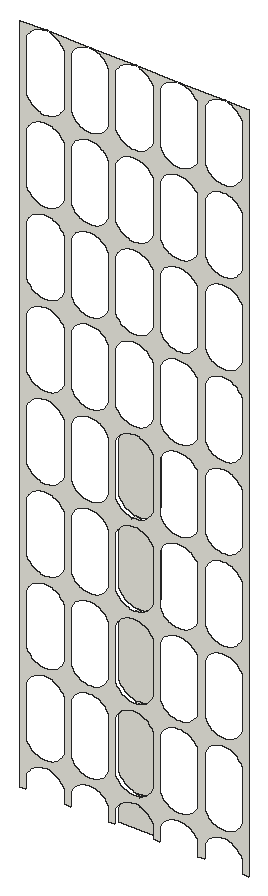
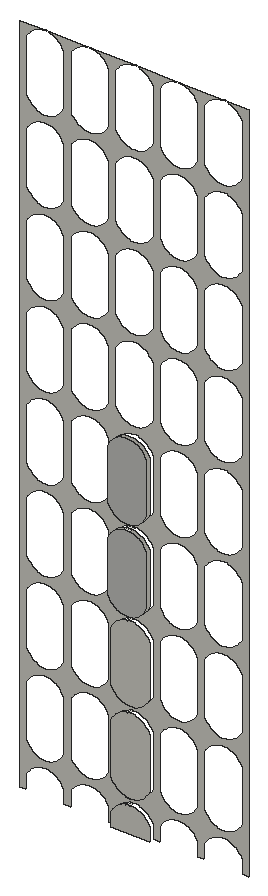
# SketchUp Ruby script. Lengths in inches.
U = 1.inch
M = Sketchup.active_model
def pt(a) = Geom::Point3d.new(a.map { |v| v * U })
def face(e, loops, mat)
  f = e.add_face(loops[0].map { |a| pt(a) })
  loops[1..].each { |l| e.add_face(l.map { |a| pt(a) }).erase! }
  f.material = f.back_material = mat if mat
  f
end
# faces: each face lists its corners as indices into pts; further lists are holes
def faces(e, pts, list, mat = nil) = list.each { |f| face(e, (f[0].is_a?(Array) ? f : [f]).map { |l| l.map { |i| pts[i] } }, mat) }
# xy, xz, yz: faces in a plane at the given z, y or x. An outline is a flat list of corners, or four numbers for a rectangle; further outlines are holes
def ring(l) = l.size == 4 ? [[l[0], l[1]], [l[2], l[1]], [l[2], l[3]], [l[0], l[3]]] : l.each_slice(2).to_a
def flat(e, list, mat, &to3) = list.each { |f| face(e, (f[0].is_a?(Array) ? f : [f]).map { |l| ring(l).map { |u, v| to3.(u, v) } }, mat) }
def xy(e, z, list, mat = nil) = flat(e, list, mat) { |x, y| [x, y, z] }
def xz(e, y, list, mat = nil) = flat(e, list, mat) { |x, z| [x, y, z] }
def yz(e, x, list, mat = nil) = flat(e, list, mat) { |y, z| [x, y, z] }
def lines(e, pts, list) = list.each { |a, b| e.add_line(pt(pts[a]), pt(pts[b])) }
# prism: a flat outline (further loops are holes) pulled along v
def prism(e, loops, v, mat = nil)
  f = face(e, loops, mat); d = Geom::Vector3d.new(v.map { |x| x * U })
  f.pushpull(f.normal.samedirection?(d) ? d.length : -d.length)
end
def box(e, o, s, mat = nil) = prism(e, [[o, [o[0] + s[0], o[1], o[2]], [o[0] + s[0], o[1] + s[1], o[2]], [o[0], o[1] + s[1], o[2]]]], [0, 0, s[2]], mat)
def at(x, y, z, deg = 0) = Geom::Transformation.translation(pt([x, y, z])) * Geom::Transformation.rotation(ORIGIN, Z_AXIS, deg.degrees)
def axes(o, x, y, z) = Geom::Transformation.new([*x, 0, *y, 0, *z, 0, *pt(o).to_a, 1])
def part(name) = M.definitions.add(name)
# library, detail: a bought-in or finely detailed component or shape, given as its bounding box
def library(name, o, s) = part(name).tap { |d| box(d.entities, o, s) }
def detail(e, o, s) = box(e.add_group.entities, o, s)
def put(e, d, t, mat = nil) = e.add_instance(d, t).tap { |i| i.material = mat if mat }
def group(e, t, mat = nil) = e.add_group.tap { |g| g.transformation = t; g.material = mat if mat }.entities
root = M.entities
M.materials.add("Tafisa-Gardenia-or-Gardenia-PM775-4K").color = [246, 245, 235]
xz(root,138,[[[64.5,6,65.5,6,65.5,8,65.637,8.288,65.801,8.56,65.991,8.816,66.205,9.051,66.441,9.265,66.697,9.454,66.97,9.618,67.258,9.753,67.558,9.861,67.867,9.938,68.182,9.984,68.5,10,68.818,9.984,69.133,9.938,69.442,9.861,69.742,9.753,70.03,9.618,70.303,9.454,70.559,9.265,70.795,9.051,71.009,8.816,71.199,8.56,71.363,8.288,71.5,8,71.5,6,72.5,6,72.5,8,72.637,8.288,72.801,8.56,72.991,8.816,73.205,9.051,73.441,9.265,73.697,9.454,73.97,9.618,74.258,9.753,74.558,9.861,74.867,9.938,75.182,9.984,75.5,10,75.818,9.984,76.133,9.938,76.442,9.861,76.742,9.753,77.03,9.618,77.303,9.454,77.559,9.265,77.795,9.051,78.009,8.816,78.199,8.56,78.363,8.288,78.5,8,78.5,6,79.5,6,79.5,8,79.637,8.288,79.801,8.56,79.991,8.816,80.205,9.051,80.441,9.265,80.697,9.454,80.97,9.618,81.258,9.753,81.558,9.861,81.867,9.938,82.182,9.984,82.5,10,82.818,9.984,83.133,9.938,83.442,9.861,83.742,9.753,84.03,9.618,84.303,9.454,84.559,9.265,84.795,9.051,85.009,8.816,85.199,8.56,85.363,8.288,85.5,8,85.5,6,86.5,6,86.5,8,86.64,8.288,86.808,8.561,87.001,8.817,87.218,9.052,87.457,9.266,87.715,9.455,87.991,9.618,88.281,9.754,88.583,9.861,88.894,9.938,89.211,9.984,89.531,10,89.851,9.984,90.168,9.938,90.479,9.861,90.781,9.754,91.071,9.618,91.347,9.455,91.606,9.266,91.845,9.052,92.062,8.817,92.255,8.561,92.422,8.288,92.5625,8,92.5625,6,93.5625,6,93.5625,8,93.696,8.287,93.857,8.559,94.043,8.815,94.255,9.05,94.488,9.264,94.741,9.453,95.012,9.617,95.298,9.753,95.596,9.86,95.902,9.9375,96.215,9.984,96.531,10,96.847,9.984,97.16,9.9375,97.467,9.86,97.765,9.753,98.05,9.617,98.321,9.453,98.574,9.264,98.808,9.05,99.019,8.815,99.206,8.559,99.367,8.287,99.5,8,99.5,6,100.5,6,100.5,114,96.531,114,96.847,113.984,97.16,113.9375,97.467,113.86,97.765,113.753,98.05,113.617,98.321,113.453,98.574,113.264,98.808,113.05,99.019,112.815,99.206,112.559,99.367,112.287,99.5,112,99.5,104,99.367,103.713,99.206,103.441,99.019,103.185,98.808,102.95,98.574,102.736,98.321,102.547,98.05,102.383,97.765,102.247,97.467,102.14,97.16,102.0625,96.847,102.016,96.531,102,96.215,102.016,95.902,102.0625,95.596,102.14,95.298,102.247,95.012,102.383,94.741,102.547,94.488,102.736,94.255,102.95,94.043,103.185,93.857,103.441,93.696,103.713,93.5625,104,93.5625,112,93.696,112.287,93.857,112.559,94.043,112.815,94.255,113.05,94.488,113.264,94.741,113.453,95.012,113.617,95.298,113.753,95.596,113.86,95.902,113.9375,96.215,113.984,96.531,114,89.531,114,89.851,113.984,90.168,113.938,90.479,113.861,90.781,113.754,91.071,113.618,91.347,113.455,91.606,113.266,91.845,113.052,92.062,112.817,92.255,112.561,92.422,112.288,92.5625,112,92.5625,104,92.422,103.712,92.255,103.439,92.062,103.183,91.845,102.948,91.606,102.734,91.347,102.545,91.071,102.382,90.781,102.246,90.479,102.139,90.168,102.062,89.851,102.016,89.531,102,89.211,102.016,88.894,102.062,88.583,102.139,88.281,102.246,87.991,102.382,87.715,102.545,87.457,102.734,87.218,102.948,87.001,103.183,86.808,103.439,86.64,103.712,86.5,104,86.5,112,86.64,112.288,86.808,112.561,87.001,112.817,87.218,113.052,87.457,113.266,87.715,113.455,87.991,113.618,88.281,113.754,88.583,113.861,88.894,113.938,89.211,113.984,89.531,114,82.5,114,82.818,113.984,83.133,113.938,83.442,113.861,83.742,113.753,84.03,113.618,84.303,113.454,84.559,113.265,84.795,113.051,85.009,112.816,85.199,112.56,85.363,112.288,85.5,112,85.5,104,85.363,103.712,85.199,103.44,85.009,103.184,84.795,102.949,84.559,102.735,84.303,102.546,84.03,102.382,83.742,102.247,83.442,102.139,83.133,102.062,82.818,102.016,82.5,102,82.182,102.016,81.867,102.062,81.558,102.139,81.258,102.247,80.97,102.382,80.697,102.546,80.441,102.735,80.205,102.949,79.991,103.184,79.801,103.44,79.637,103.712,79.5,104,79.5,112,79.637,112.288,79.801,112.56,79.991,112.816,80.205,113.051,80.441,113.265,80.697,113.454,80.97,113.618,81.258,113.753,81.558,113.861,81.867,113.938,82.182,113.984,82.5,114,75.5,114,75.818,113.984,76.133,113.938,76.442,113.861,76.742,113.753,77.03,113.618,77.303,113.454,77.559,113.265,77.795,113.051,78.009,112.816,78.199,112.56,78.363,112.288,78.5,112,78.5,104,78.363,103.712,78.199,103.44,78.009,103.184,77.795,102.949,77.559,102.735,77.303,102.546,77.03,102.382,76.742,102.247,76.442,102.139,76.133,102.062,75.818,102.016,75.5,102,75.182,102.016,74.867,102.062,74.558,102.139,74.258,102.247,73.97,102.382,73.697,102.546,73.441,102.735,73.205,102.949,72.991,103.184,72.801,103.44,72.637,103.712,72.5,104,72.5,112,72.637,112.288,72.801,112.56,72.991,112.816,73.205,113.051,73.441,113.265,73.697,113.454,73.97,113.618,74.258,113.753,74.558,113.861,74.867,113.938,75.182,113.984,75.5,114,68.5,114,68.818,113.984,69.133,113.938,69.442,113.861,69.742,113.753,70.03,113.618,70.303,113.454,70.559,113.265,70.795,113.051,71.009,112.816,71.199,112.56,71.363,112.288,71.5,112,71.5,104,71.363,103.712,71.199,103.44,71.009,103.184,70.795,102.949,70.559,102.735,70.303,102.546,70.03,102.382,69.742,102.247,69.442,102.139,69.133,102.062,68.818,102.016,68.5,102,68.182,102.016,67.867,102.062,67.558,102.139,67.258,102.247,66.97,102.382,66.697,102.546,66.441,102.735,66.205,102.949,65.991,103.184,65.801,103.44,65.637,103.712,65.5,104,65.5,112,65.637,112.288,65.801,112.56,65.991,112.816,66.205,113.051,66.441,113.265,66.697,113.454,66.97,113.618,67.258,113.753,67.558,113.861,67.867,113.938,68.182,113.984,68.5,114,64.5,114],[89.531,89,89.211,89.016,88.894,89.062,88.583,89.139,88.281,89.246,87.991,89.382,87.715,89.545,87.457,89.734,87.218,89.948,87.001,90.183,86.808,90.439,86.64,90.712,86.5,91,86.5,99,86.64,99.288,86.808,99.561,87.001,99.817,87.218,100.052,87.457,100.266,87.715,100.455,87.991,100.618,88.281,100.754,88.583,100.861,88.894,100.938,89.211,100.984,89.531,101,89.851,100.984,90.168,100.938,90.479,100.861,90.781,100.754,91.071,100.618,91.347,100.455,91.606,100.266,91.845,100.052,92.062,99.817,92.255,99.561,92.422,99.288,92.5625,99,92.5625,91,92.422,90.712,92.255,90.439,92.062,90.183,91.845,89.948,91.606,89.734,91.347,89.545,91.071,89.382,90.781,89.246,90.479,89.139,90.168,89.062,89.851,89.016],[89.531,11,89.211,11.016,88.894,11.062,88.583,11.139,88.281,11.246,87.991,11.382,87.715,11.545,87.457,11.734,87.218,11.948,87.001,12.183,86.808,12.439,86.64,12.712,86.5,13,86.5,21,86.64,21.288,86.808,21.561,87.001,21.817,87.218,22.052,87.457,22.266,87.715,22.455,87.991,22.618,88.281,22.754,88.583,22.861,88.894,22.938,89.016,22.956,89.211,22.984,89.531,23,89.851,22.984,90.168,22.938,90.479,22.861,90.781,22.754,91.071,22.618,91.347,22.455,91.606,22.266,91.845,22.052,92.062,21.817,92.255,21.561,92.422,21.288,92.5625,21,92.5625,13,92.422,12.712,92.255,12.439,92.062,12.183,91.845,11.948,91.606,11.734,91.347,11.545,91.071,11.382,90.781,11.246,90.479,11.139,90.168,11.062,89.851,11.016],[89.531,24,89.211,24.016,89.016,24.044,88.894,24.062,88.583,24.139,88.281,24.246,87.991,24.382,87.715,24.545,87.457,24.734,87.218,24.948,87.001,25.183,86.808,25.439,86.64,25.712,86.5,26,86.5,34,86.64,34.288,86.808,34.561,86.863,34.634,87.001,34.817,87.218,35.052,87.457,35.266,87.715,35.455,87.991,35.618,88.281,35.754,88.583,35.861,88.894,35.938,89.016,35.956,89.211,35.984,89.531,36,89.851,35.984,90.168,35.938,90.479,35.861,90.781,35.754,91.071,35.618,91.347,35.455,91.606,35.266,91.845,35.052,92.062,34.817,92.255,34.561,92.422,34.288,92.5625,34,92.5625,26,92.422,25.712,92.255,25.439,92.062,25.183,91.845,24.948,91.606,24.734,91.347,24.545,91.071,24.382,90.781,24.246,90.479,24.139,90.168,24.062,89.851,24.016],[89.531,76,89.211,76.016,89.016,76.044,88.894,76.062,88.583,76.139,88.281,76.246,87.991,76.382,87.715,76.545,87.457,76.734,87.218,76.948,87.001,77.183,86.808,77.439,86.64,77.712,86.5,78,86.5,86,86.64,86.288,86.808,86.561,87.001,86.817,87.218,87.052,87.457,87.266,87.715,87.455,87.991,87.618,88.281,87.754,88.583,87.861,88.894,87.938,89.211,87.984,89.531,88,89.851,87.984,90.168,87.938,90.479,87.861,90.781,87.754,91.071,87.618,91.347,87.455,91.606,87.266,91.845,87.052,92.062,86.817,92.255,86.561,92.422,86.288,92.5625,86,92.5625,78,92.422,77.712,92.255,77.439,92.062,77.183,91.845,76.948,91.606,76.734,91.347,76.545,91.071,76.382,90.781,76.246,90.479,76.139,90.168,76.062,89.851,76.016],[89.531,63,89.211,63.016,89.016,63.044,88.894,63.062,88.782,63.09,88.583,63.139,88.281,63.246,87.991,63.382,87.715,63.545,87.457,63.734,87.218,63.948,87.001,64.183,86.808,64.439,86.64,64.712,86.5,65,86.5,73,86.64,73.288,86.808,73.561,87.001,73.817,87.218,74.052,87.457,74.266,87.715,74.455,87.991,74.618,88.281,74.754,88.583,74.861,88.894,74.938,89.016,74.956,89.211,74.984,89.531,75,89.851,74.984,90.168,74.938,90.479,74.861,90.781,74.754,91.071,74.618,91.347,74.455,91.606,74.266,91.845,74.052,92.062,73.817,92.255,73.561,92.422,73.288,92.5625,73,92.5625,65,92.422,64.712,92.255,64.439,92.062,64.183,91.845,63.948,91.606,63.734,91.347,63.545,91.071,63.382,90.781,63.246,90.479,63.139,90.168,63.062,89.851,63.016],[89.531,50,89.211,50.016,89.016,50.044,88.894,50.062,88.583,50.139,88.281,50.246,87.991,50.382,87.715,50.545,87.457,50.734,87.218,50.948,87.001,51.183,86.808,51.439,86.64,51.712,86.5,52,86.5,60,86.64,60.288,86.808,60.561,87.001,60.817,87.218,61.052,87.457,61.266,87.715,61.455,87.991,61.618,88.281,61.754,88.583,61.861,88.894,61.938,89.016,61.956,89.211,61.984,89.531,62,89.851,61.984,90.168,61.938,90.479,61.861,90.781,61.754,91.071,61.618,91.347,61.455,91.606,61.266,91.845,61.052,92.062,60.817,92.255,60.561,92.422,60.288,92.5625,60,92.5625,52,92.422,51.712,92.255,51.439,92.062,51.183,91.845,50.948,91.606,50.734,91.347,50.545,91.071,50.382,90.781,50.246,90.479,50.139,90.168,50.062,89.851,50.016],[89.531,37,89.211,37.016,89.016,37.044,88.894,37.062,88.583,37.139,88.281,37.246,87.991,37.382,87.715,37.545,87.457,37.734,87.218,37.948,87.001,38.183,86.808,38.439,86.64,38.712,86.5,39,86.5,47,86.64,47.288,86.808,47.561,87.001,47.817,87.218,48.052,87.457,48.266,87.715,48.455,87.991,48.618,88.281,48.754,88.583,48.861,88.894,48.938,89.016,48.956,89.211,48.984,89.531,49,89.851,48.984,90.168,48.938,90.479,48.861,90.781,48.754,91.071,48.618,91.347,48.455,91.606,48.266,91.845,48.052,92.062,47.817,92.255,47.561,92.422,47.288,92.5625,47,92.5625,39,92.422,38.712,92.255,38.439,92.062,38.183,91.845,37.948,91.606,37.734,91.347,37.545,91.071,37.382,90.781,37.246,90.479,37.139,90.168,37.062,89.851,37.016],[68.5,11,68.182,11.016,67.867,11.062,67.558,11.139,67.258,11.247,66.97,11.382,66.697,11.546,66.441,11.735,66.205,11.949,65.991,12.184,65.801,12.44,65.637,12.712,65.5,13,65.5,21,65.637,21.288,65.801,21.56,65.991,21.816,66.205,22.051,66.441,22.265,66.697,22.454,66.97,22.618,67.258,22.753,67.558,22.861,67.867,22.938,68.182,22.984,68.5,23,68.818,22.984,69.133,22.938,69.442,22.861,69.742,22.753,70.03,22.618,70.303,22.454,70.559,22.265,70.795,22.051,71.009,21.816,71.199,21.56,71.363,21.288,71.5,21,71.5,13,71.363,12.712,71.199,12.44,71.009,12.184,70.795,11.949,70.559,11.735,70.303,11.546,70.03,11.382,69.742,11.247,69.442,11.139,69.133,11.062,68.818,11.016],[82.5,11,82.182,11.016,81.867,11.062,81.558,11.139,81.258,11.247,80.97,11.382,80.697,11.546,80.441,11.735,80.205,11.949,79.991,12.184,79.801,12.44,79.637,12.712,79.5,13,79.5,21,79.637,21.288,79.801,21.56,79.991,21.816,80.205,22.051,80.441,22.265,80.697,22.454,80.97,22.618,81.258,22.753,81.558,22.861,81.867,22.938,82.182,22.984,82.5,23,82.818,22.984,83.133,22.938,83.442,22.861,83.742,22.753,84.03,22.618,84.303,22.454,84.559,22.265,84.795,22.051,85.009,21.816,85.199,21.56,85.363,21.288,85.5,21,85.5,13,85.363,12.712,85.199,12.44,85.009,12.184,84.795,11.949,84.559,11.735,84.303,11.546,84.03,11.382,83.742,11.247,83.442,11.139,83.133,11.062,82.818,11.016],[75.5,11,75.182,11.016,74.867,11.062,74.558,11.139,74.258,11.247,73.97,11.382,73.697,11.546,73.441,11.735,73.205,11.949,72.991,12.184,72.801,12.44,72.637,12.712,72.5,13,72.5,21,72.637,21.288,72.801,21.56,72.991,21.816,73.205,22.051,73.441,22.265,73.697,22.454,73.97,22.618,74.258,22.753,74.558,22.861,74.867,22.938,75.182,22.984,75.5,23,75.818,22.984,76.133,22.938,76.442,22.861,76.742,22.753,77.03,22.618,77.303,22.454,77.559,22.265,77.795,22.051,78.009,21.816,78.199,21.56,78.363,21.288,78.5,21,78.5,13,78.363,12.712,78.199,12.44,78.009,12.184,77.795,11.949,77.559,11.735,77.303,11.546,77.03,11.382,76.742,11.247,76.442,11.139,76.133,11.062,75.818,11.016],[68.5,50,68.182,50.016,67.867,50.062,67.558,50.139,67.258,50.247,66.97,50.382,66.697,50.546,66.441,50.735,66.205,50.949,65.991,51.184,65.801,51.44,65.637,51.712,65.5,52,65.5,60,65.637,60.288,65.801,60.56,65.991,60.816,66.205,61.051,66.441,61.265,66.697,61.454,66.97,61.618,67.258,61.753,67.558,61.861,67.867,61.938,68.182,61.984,68.5,62,68.818,61.984,69.133,61.938,69.442,61.861,69.742,61.753,70.03,61.618,70.303,61.454,70.559,61.265,70.795,61.051,71.009,60.816,71.199,60.56,71.363,60.288,71.5,60,71.5,52,71.363,51.712,71.199,51.44,71.009,51.184,70.795,50.949,70.559,50.735,70.303,50.546,70.03,50.382,69.742,50.247,69.442,50.139,69.133,50.062,68.818,50.016],[82.5,63,82.182,63.016,81.867,63.062,81.558,63.139,81.258,63.247,80.97,63.382,80.697,63.546,80.441,63.735,80.205,63.949,79.991,64.184,79.801,64.44,79.637,64.712,79.5,65,79.5,73,79.637,73.288,79.801,73.56,79.991,73.816,80.205,74.051,80.441,74.265,80.697,74.454,80.97,74.618,81.258,74.753,81.558,74.861,81.867,74.938,82.182,74.984,82.5,75,82.818,74.984,83.133,74.938,83.442,74.861,83.742,74.753,84.03,74.618,84.303,74.454,84.559,74.265,84.795,74.051,85.009,73.816,85.199,73.56,85.363,73.288,85.5,73,85.5,65,85.363,64.712,85.199,64.44,85.009,64.184,84.795,63.949,84.559,63.735,84.303,63.546,84.03,63.382,83.742,63.247,83.442,63.139,83.133,63.062,82.818,63.016],[75.5,63,75.182,63.016,74.867,63.062,74.558,63.139,74.258,63.247,73.97,63.382,73.697,63.546,73.441,63.735,73.205,63.949,72.991,64.184,72.801,64.44,72.637,64.712,72.5,65,72.5,73,72.637,73.288,72.801,73.56,72.991,73.816,73.205,74.051,73.441,74.265,73.697,74.454,73.97,74.618,74.258,74.753,74.558,74.861,74.867,74.938,75.182,74.984,75.5,75,75.818,74.984,76.133,74.938,76.442,74.861,76.742,74.753,77.03,74.618,77.303,74.454,77.559,74.265,77.795,74.051,78.009,73.816,78.199,73.56,78.363,73.288,78.5,73,78.5,65,78.363,64.712,78.199,64.44,78.009,64.184,77.795,63.949,77.559,63.735,77.303,63.546,77.03,63.382,76.742,63.247,76.442,63.139,76.133,63.062,75.818,63.016],[82.5,89,82.182,89.016,81.867,89.062,81.558,89.139,81.258,89.247,80.97,89.382,80.697,89.546,80.441,89.735,80.205,89.949,79.991,90.184,79.801,90.44,79.637,90.712,79.5,91,79.5,99,79.637,99.288,79.801,99.56,79.991,99.816,80.205,100.051,80.441,100.265,80.697,100.454,80.97,100.618,81.258,100.753,81.558,100.861,81.867,100.938,82.182,100.984,82.5,101,82.818,100.984,83.133,100.938,83.442,100.861,83.742,100.753,84.03,100.618,84.303,100.454,84.559,100.265,84.795,100.051,85.009,99.816,85.199,99.56,85.363,99.288,85.5,99,85.5,91,85.363,90.712,85.199,90.44,85.009,90.184,84.795,89.949,84.559,89.735,84.303,89.546,84.03,89.382,83.742,89.247,83.442,89.139,83.133,89.062,82.818,89.016],[75.5,89,75.182,89.016,74.867,89.062,74.558,89.139,74.258,89.247,73.97,89.382,73.697,89.546,73.441,89.735,73.205,89.949,72.991,90.184,72.801,90.44,72.637,90.712,72.5,91,72.5,99,72.637,99.288,72.801,99.56,72.991,99.816,73.205,100.051,73.441,100.265,73.697,100.454,73.97,100.618,74.258,100.753,74.558,100.861,74.867,100.938,75.182,100.984,75.5,101,75.818,100.984,76.133,100.938,76.442,100.861,76.742,100.753,77.03,100.618,77.303,100.454,77.559,100.265,77.795,100.051,78.009,99.816,78.199,99.56,78.363,99.288,78.5,99,78.5,91,78.363,90.712,78.199,90.44,78.009,90.184,77.795,89.949,77.559,89.735,77.303,89.546,77.03,89.382,76.742,89.247,76.442,89.139,76.133,89.062,75.818,89.016],[68.5,24,68.182,24.016,67.867,24.062,67.558,24.139,67.258,24.247,66.97,24.382,66.697,24.546,66.441,24.735,66.205,24.949,65.991,25.184,65.801,25.44,65.637,25.712,65.5,26,65.5,34,65.637,34.288,65.801,34.56,65.991,34.816,66.205,35.051,66.441,35.265,66.697,35.454,66.97,35.618,67.258,35.753,67.558,35.861,67.867,35.938,68.182,35.984,68.5,36,68.818,35.984,69.133,35.938,69.442,35.861,69.742,35.753,70.03,35.618,70.303,35.454,70.559,35.265,70.795,35.051,71.009,34.816,71.199,34.56,71.363,34.288,71.5,34,71.5,26,71.363,25.712,71.199,25.44,71.009,25.184,70.795,24.949,70.559,24.735,70.303,24.546,70.03,24.382,69.742,24.247,69.442,24.139,69.133,24.062,68.818,24.016],[75.5,24,75.182,24.016,74.867,24.062,74.558,24.139,74.258,24.247,73.97,24.382,73.697,24.546,73.441,24.735,73.205,24.949,72.991,25.184,72.801,25.44,72.637,25.712,72.5,26,72.5,34,72.637,34.288,72.801,34.56,72.991,34.816,73.205,35.051,73.441,35.265,73.697,35.454,73.97,35.618,74.258,35.753,74.558,35.861,74.867,35.938,75.182,35.984,75.5,36,75.818,35.984,76.133,35.938,76.442,35.861,76.742,35.753,77.03,35.618,77.303,35.454,77.559,35.265,77.795,35.051,78.009,34.816,78.199,34.56,78.363,34.288,78.5,34,78.5,26,78.363,25.712,78.199,25.44,78.009,25.184,77.795,24.949,77.559,24.735,77.303,24.546,77.03,24.382,76.742,24.247,76.442,24.139,76.133,24.062,75.818,24.016],[82.5,24,82.182,24.016,81.867,24.062,81.558,24.139,81.258,24.247,80.97,24.382,80.697,24.546,80.441,24.735,80.205,24.949,79.991,25.184,79.801,25.44,79.637,25.712,79.5,26,79.5,34,79.637,34.288,79.801,34.56,79.991,34.816,80.205,35.051,80.441,35.265,80.697,35.454,80.97,35.618,81.258,35.753,81.558,35.861,81.867,35.938,82.182,35.984,82.5,36,82.818,35.984,83.133,35.938,83.442,35.861,83.742,35.753,84.03,35.618,84.303,35.454,84.559,35.265,84.795,35.051,85.009,34.816,85.199,34.56,85.363,34.288,85.5,34,85.5,26,85.363,25.712,85.199,25.44,85.009,25.184,84.795,24.949,84.559,24.735,84.303,24.546,84.03,24.382,83.742,24.247,83.442,24.139,83.133,24.062,82.818,24.016],[75.5,37,75.182,37.016,74.867,37.062,74.558,37.139,74.258,37.247,73.97,37.382,73.697,37.546,73.441,37.735,73.205,37.949,72.991,38.184,72.801,38.44,72.637,38.712,72.5,39,72.5,47,72.637,47.288,72.801,47.56,72.991,47.816,73.205,48.051,73.441,48.265,73.697,48.454,73.97,48.618,74.258,48.753,74.558,48.861,74.867,48.938,75.182,48.984,75.5,49,75.818,48.984,76.133,48.938,76.442,48.861,76.742,48.753,77.03,48.618,77.303,48.454,77.559,48.265,77.795,48.051,78.009,47.816,78.199,47.56,78.363,47.288,78.5,47,78.5,39,78.363,38.712,78.199,38.44,78.009,38.184,77.795,37.949,77.559,37.735,77.303,37.546,77.03,37.382,76.742,37.247,76.442,37.139,76.133,37.062,75.818,37.016],[68.5,37,68.182,37.016,67.867,37.062,67.558,37.139,67.258,37.247,66.97,37.382,66.697,37.546,66.441,37.735,66.205,37.949,65.991,38.184,65.801,38.44,65.637,38.712,65.5,39,65.5,47,65.637,47.288,65.801,47.56,65.991,47.816,66.205,48.051,66.441,48.265,66.697,48.454,66.97,48.618,67.258,48.753,67.558,48.861,67.867,48.938,68.182,48.984,68.5,49,68.818,48.984,69.133,48.938,69.442,48.861,69.742,48.753,70.03,48.618,70.303,48.454,70.559,48.265,70.795,48.051,71.009,47.816,71.199,47.56,71.363,47.288,71.5,47,71.5,39,71.363,38.712,71.199,38.44,71.009,38.184,70.795,37.949,70.559,37.735,70.303,37.546,70.03,37.382,69.742,37.247,69.442,37.139,69.133,37.062,68.818,37.016],[75.5,50,75.182,50.016,74.867,50.062,74.558,50.139,74.258,50.247,73.97,50.382,73.697,50.546,73.441,50.735,73.205,50.949,72.991,51.184,72.801,51.44,72.637,51.712,72.5,52,72.5,60,72.637,60.288,72.801,60.56,72.991,60.816,73.205,61.051,73.441,61.265,73.697,61.454,73.97,61.618,74.258,61.753,74.558,61.861,74.867,61.938,75.182,61.984,75.5,62,75.818,61.984,76.133,61.938,76.442,61.861,76.742,61.753,77.03,61.618,77.303,61.454,77.559,61.265,77.795,61.051,78.009,60.816,78.199,60.56,78.363,60.288,78.5,60,78.5,52,78.363,51.712,78.199,51.44,78.009,51.184,77.795,50.949,77.559,50.735,77.303,50.546,77.03,50.382,76.742,50.247,76.442,50.139,76.133,50.062,75.818,50.016],[68.5,63,68.182,63.016,67.867,63.062,67.558,63.139,67.258,63.247,66.97,63.382,66.697,63.546,66.441,63.735,66.205,63.949,65.991,64.184,65.801,64.44,65.637,64.712,65.5,65,65.5,73,65.637,73.288,65.801,73.56,65.991,73.816,66.205,74.051,66.441,74.265,66.697,74.454,66.97,74.618,67.258,74.753,67.558,74.861,67.867,74.938,68.182,74.984,68.5,75,68.818,74.984,69.133,74.938,69.442,74.861,69.742,74.753,70.03,74.618,70.303,74.454,70.559,74.265,70.795,74.051,71.009,73.816,71.199,73.56,71.363,73.288,71.5,73,71.5,65,71.363,64.712,71.199,64.44,71.009,64.184,70.795,63.949,70.559,63.735,70.303,63.546,70.03,63.382,69.742,63.247,69.442,63.139,69.133,63.062,68.818,63.016],[82.5,76,82.182,76.016,81.867,76.062,81.558,76.139,81.258,76.247,80.97,76.382,80.697,76.546,80.441,76.735,80.205,76.949,79.991,77.184,79.801,77.44,79.637,77.712,79.5,78,79.5,86,79.637,86.288,79.801,86.56,79.991,86.816,80.205,87.051,80.441,87.265,80.697,87.454,80.97,87.618,81.258,87.753,81.558,87.861,81.867,87.938,82.182,87.984,82.5,88,82.818,87.984,83.133,87.938,83.442,87.861,83.742,87.753,84.03,87.618,84.303,87.454,84.559,87.265,84.795,87.051,85.009,86.816,85.199,86.56,85.363,86.288,85.5,86,85.5,78,85.363,77.712,85.199,77.44,85.009,77.184,84.795,76.949,84.559,76.735,84.303,76.546,84.03,76.382,83.742,76.247,83.442,76.139,83.133,76.062,82.818,76.016],[75.5,76,75.182,76.016,74.867,76.062,74.558,76.139,74.258,76.247,73.97,76.382,73.697,76.546,73.441,76.735,73.205,76.949,72.991,77.184,72.801,77.44,72.637,77.712,72.5,78,72.5,86,72.637,86.288,72.801,86.56,72.991,86.816,73.205,87.051,73.441,87.265,73.697,87.454,73.97,87.618,74.258,87.753,74.558,87.861,74.867,87.938,75.182,87.984,75.5,88,75.818,87.984,76.133,87.938,76.442,87.861,76.742,87.753,77.03,87.618,77.303,87.454,77.559,87.265,77.795,87.051,78.009,86.816,78.199,86.56,78.363,86.288,78.5,86,78.5,78,78.363,77.712,78.199,77.44,78.009,77.184,77.795,76.949,77.559,76.735,77.303,76.546,77.03,76.382,76.742,76.247,76.442,76.139,76.133,76.062,75.818,76.016],[68.5,76,68.182,76.016,67.867,76.062,67.558,76.139,67.258,76.247,66.97,76.382,66.697,76.546,66.441,76.735,66.205,76.949,65.991,77.184,65.801,77.44,65.637,77.712,65.5,78,65.5,86,65.637,86.288,65.801,86.56,65.991,86.816,66.205,87.051,66.441,87.265,66.697,87.454,66.97,87.618,67.258,87.753,67.558,87.861,67.867,87.938,68.182,87.984,68.5,88,68.818,87.984,69.133,87.938,69.442,87.861,69.742,87.753,70.03,87.618,70.303,87.454,70.559,87.265,70.795,87.051,71.009,86.816,71.199,86.56,71.363,86.288,71.5,86,71.5,78,71.363,77.712,71.199,77.44,71.009,77.184,70.795,76.949,70.559,76.735,70.303,76.546,70.03,76.382,69.742,76.247,69.442,76.139,69.133,76.062,68.818,76.016],[68.5,89,68.182,89.016,67.867,89.062,67.558,89.139,67.258,89.247,66.97,89.382,66.697,89.546,66.441,89.735,66.205,89.949,65.991,90.184,65.801,90.44,65.637,90.712,65.5,91,65.5,99,65.637,99.288,65.801,99.56,65.991,99.816,66.205,100.051,66.441,100.265,66.697,100.454,66.97,100.618,67.258,100.753,67.558,100.861,67.867,100.938,68.182,100.984,68.5,101,68.818,100.984,69.133,100.938,69.442,100.861,69.742,100.753,70.03,100.618,70.303,100.454,70.559,100.265,70.795,100.051,71.009,99.816,71.199,99.56,71.363,99.288,71.5,99,71.5,91,71.363,90.712,71.199,90.44,71.009,90.184,70.795,89.949,70.559,89.735,70.303,89.546,70.03,89.382,69.742,89.247,69.442,89.139,69.133,89.062,68.818,89.016],[82.5,50,82.182,50.016,81.867,50.062,81.558,50.139,81.557,50.14,81.258,50.247,80.97,50.382,80.697,50.546,80.441,50.735,80.205,50.949,79.991,51.184,79.801,51.44,79.637,51.712,79.5,52,79.5,60,79.637,60.288,79.801,60.56,79.991,60.816,80.205,61.051,80.441,61.265,80.697,61.454,80.97,61.618,81.258,61.753,81.558,61.861,81.867,61.938,82.182,61.984,82.5,62,82.818,61.984,83.133,61.938,83.442,61.861,83.742,61.753,84.03,61.618,84.303,61.454,84.559,61.265,84.795,61.051,85.009,60.816,85.199,60.56,85.363,60.288,85.5,60,85.5,52,85.363,51.712,85.199,51.44,85.009,51.184,84.795,50.949,84.559,50.735,84.303,50.546,84.03,50.382,83.742,50.247,83.442,50.139,83.133,50.062,82.818,50.016],[82.5,37,82.182,37.016,81.867,37.062,81.558,37.139,81.258,37.247,80.97,37.382,80.697,37.546,80.441,37.735,80.205,37.949,79.991,38.184,79.801,38.44,79.637,38.712,79.5,39,79.5,47,79.637,47.288,79.801,47.56,79.991,47.816,80.205,48.051,80.441,48.265,80.697,48.454,80.97,48.618,81.258,48.753,81.457,48.824,81.558,48.861,81.867,48.938,82.182,48.984,82.5,49,82.818,48.984,83.133,48.938,83.442,48.861,83.742,48.753,84.03,48.618,84.303,48.454,84.559,48.265,84.795,48.051,85.009,47.816,85.199,47.56,85.363,47.288,85.5,47,85.5,39,85.363,38.712,85.199,38.44,85.009,38.184,84.795,37.949,84.559,37.735,84.457,37.66,84.303,37.546,84.03,37.382,83.742,37.247,83.442,37.139,83.133,37.062,82.818,37.016],[96.531,24,96.215,24.016,95.902,24.0625,95.596,24.14,95.298,24.247,95.012,24.383,94.741,24.547,94.488,24.736,94.255,24.95,94.043,25.185,93.857,25.441,93.696,25.713,93.5625,26,93.5625,34,93.696,34.287,93.857,34.559,94.043,34.815,94.255,35.05,94.488,35.264,94.741,35.453,95.012,35.617,95.298,35.753,95.596,35.86,95.902,35.9375,96.215,35.984,96.531,36,96.847,35.984,97.16,35.9375,97.467,35.86,97.765,35.753,98.05,35.617,98.321,35.453,98.574,35.264,98.808,35.05,99.019,34.815,99.206,34.559,99.367,34.287,99.5,34,99.5,26,99.367,25.713,99.206,25.441,99.019,25.185,98.808,24.95,98.574,24.736,98.321,24.547,98.05,24.383,97.765,24.247,97.467,24.14,97.16,24.0625,96.847,24.016],[96.531,11,96.215,11.016,95.902,11.0625,95.596,11.14,95.298,11.247,95.012,11.383,94.741,11.547,94.488,11.736,94.255,11.95,94.043,12.185,93.857,12.441,93.696,12.713,93.5625,13,93.5625,21,93.696,21.287,93.857,21.559,94.043,21.815,94.255,22.05,94.488,22.264,94.741,22.453,95.012,22.617,95.298,22.753,95.596,22.86,95.902,22.9375,96.215,22.984,96.531,23,96.847,22.984,97.16,22.9375,97.467,22.86,97.765,22.753,98.05,22.617,98.321,22.453,98.574,22.264,98.808,22.05,99.019,21.815,99.206,21.559,99.367,21.287,99.5,21,99.5,13,99.367,12.713,99.206,12.441,99.019,12.185,98.808,11.95,98.574,11.736,98.321,11.547,98.05,11.383,97.765,11.247,97.467,11.14,97.16,11.0625,96.847,11.016],[96.531,37,96.215,37.016,95.902,37.0625,95.596,37.14,95.298,37.247,95.012,37.383,94.741,37.547,94.488,37.736,94.255,37.95,94.043,38.185,93.857,38.441,93.696,38.713,93.5625,39,93.5625,47,93.696,47.287,93.857,47.559,94.043,47.815,94.255,48.05,94.488,48.264,94.741,48.453,95.012,48.617,95.298,48.753,95.596,48.86,95.902,48.9375,96.215,48.984,96.531,49,96.847,48.984,97.16,48.9375,97.467,48.86,97.765,48.753,98.05,48.617,98.321,48.453,98.574,48.264,98.808,48.05,99.019,47.815,99.206,47.559,99.367,47.287,99.5,47,99.5,39,99.367,38.713,99.206,38.441,99.019,38.185,98.808,37.95,98.574,37.736,98.321,37.547,98.05,37.383,97.765,37.247,97.467,37.14,97.16,37.0625,96.847,37.016],[96.531,50,96.215,50.016,95.902,50.0625,95.596,50.14,95.298,50.247,95.012,50.383,94.741,50.547,94.488,50.736,94.255,50.95,94.043,51.185,93.857,51.441,93.696,51.713,93.5625,52,93.5625,60,93.696,60.287,93.857,60.559,94.043,60.815,94.255,61.05,94.488,61.264,94.741,61.453,95.012,61.617,95.298,61.753,95.596,61.86,95.902,61.9375,96.215,61.984,96.531,62,96.847,61.984,97.16,61.9375,97.467,61.86,97.765,61.753,98.05,61.617,98.321,61.453,98.574,61.264,98.808,61.05,99.019,60.815,99.206,60.559,99.367,60.287,99.5,60,99.5,52,99.367,51.713,99.206,51.441,99.019,51.185,98.808,50.95,98.574,50.736,98.321,50.547,98.05,50.383,97.765,50.247,97.467,50.14,97.16,50.0625,96.847,50.016],[96.531,89,96.215,89.016,95.902,89.0625,95.596,89.14,95.298,89.247,95.012,89.383,94.741,89.547,94.488,89.736,94.255,89.95,94.043,90.185,93.857,90.441,93.696,90.713,93.5625,91,93.5625,99,93.696,99.287,93.857,99.559,94.043,99.815,94.255,100.05,94.488,100.264,94.741,100.453,95.012,100.617,95.298,100.753,95.596,100.86,95.902,100.9375,96.215,100.984,96.531,101,96.847,100.984,97.16,100.9375,97.467,100.86,97.765,100.753,98.05,100.617,98.321,100.453,98.574,100.264,98.808,100.05,99.019,99.815,99.206,99.559,99.367,99.287,99.5,99,99.5,91,99.367,90.713,99.206,90.441,99.019,90.185,98.808,89.95,98.574,89.736,98.321,89.547,98.05,89.383,97.765,89.247,97.467,89.14,97.16,89.0625,96.847,89.016],[96.531,76,96.215,76.016,95.902,76.0625,95.596,76.14,95.298,76.247,95.012,76.383,94.741,76.547,94.488,76.736,94.255,76.95,94.043,77.185,93.857,77.441,93.696,77.713,93.5625,78,93.5625,86,93.696,86.287,93.857,86.559,94.043,86.815,94.255,87.05,94.488,87.264,94.741,87.453,95.012,87.617,95.298,87.753,95.596,87.86,95.902,87.9375,96.215,87.984,96.531,88,96.847,87.984,97.16,87.9375,97.467,87.86,97.765,87.753,98.05,87.617,98.321,87.453,98.574,87.264,98.808,87.05,99.019,86.815,99.206,86.559,99.367,86.287,99.5,86,99.5,78,99.367,77.713,99.206,77.441,99.019,77.185,98.808,76.95,98.574,76.736,98.321,76.547,98.05,76.383,97.765,76.247,97.467,76.14,97.16,76.0625,96.847,76.016],[96.531,63,96.215,63.016,95.902,63.0625,95.596,63.14,95.298,63.247,95.012,63.383,94.741,63.547,94.488,63.736,94.255,63.95,94.043,64.185,93.857,64.441,93.696,64.713,93.5625,65,93.5625,73,93.696,73.287,93.857,73.559,94.043,73.815,94.255,74.05,94.488,74.264,94.741,74.453,95.012,74.617,95.298,74.753,95.596,74.86,95.902,74.9375,96.215,74.984,96.531,75,96.847,74.984,97.16,74.9375,97.467,74.86,97.765,74.753,98.05,74.617,98.321,74.453,98.574,74.264,98.808,74.05,99.019,73.815,99.206,73.559,99.367,73.287,99.5,73,99.5,65,99.367,64.713,99.206,64.441,99.019,64.185,98.808,63.95,98.574,63.736,98.321,63.547,98.05,63.383,97.765,63.247,97.467,63.14,97.16,63.0625,96.847,63.016]]],"Tafisa-Gardenia-or-Gardenia-PM775-4K")
xz(root,138.787,[[79.5,6,85.5,6,85.5,8,85.363,8.288,85.199,8.56,85.009,8.816,84.795,9.051,84.559,9.265,84.303,9.454,84.03,9.618,83.742,9.753,83.442,9.861,83.133,9.938,82.818,9.984,82.5,10,82.182,9.984,81.867,9.938,81.558,9.861,81.258,9.753,80.97,9.618,80.697,9.454,80.441,9.265,80.205,9.051,79.991,8.816,79.801,8.56,79.637,8.288,79.5,8],[82.5,11,82.818,11.016,83.133,11.062,83.442,11.139,83.742,11.247,84.03,11.382,84.303,11.546,84.559,11.735,84.795,11.949,85.009,12.184,85.199,12.44,85.363,12.712,85.5,13,85.5,21,85.363,21.288,85.199,21.56,85.009,21.816,84.795,22.051,84.559,22.265,84.303,22.454,84.03,22.618,83.742,22.753,83.442,22.861,83.133,22.938,82.818,22.984,82.5,23,82.182,22.984,81.867,22.938,81.558,22.861,81.258,22.753,80.97,22.618,80.697,22.454,80.441,22.265,80.205,22.051,79.991,21.816,79.801,21.56,79.637,21.288,79.5,21,79.5,13,79.637,12.712,79.801,12.44,79.991,12.184,80.205,11.949,80.441,11.735,80.697,11.546,80.97,11.382,81.258,11.247,81.558,11.139,81.867,11.062,82.182,11.016],[82.5,24,82.818,24.016,83.133,24.062,83.442,24.139,83.742,24.247,84.03,24.382,84.303,24.546,84.559,24.735,84.795,24.949,85.009,25.184,85.199,25.44,85.363,25.712,85.5,26,85.5,34,85.363,34.288,85.199,34.56,85.009,34.816,84.795,35.051,84.559,35.265,84.303,35.454,84.03,35.618,83.742,35.753,83.442,35.861,83.133,35.938,82.818,35.984,82.5,36,82.182,35.984,81.867,35.938,81.558,35.861,81.258,35.753,80.97,35.618,80.697,35.454,80.441,35.265,80.205,35.051,79.991,34.816,79.801,34.56,79.637,34.288,79.5,34,79.5,26,79.637,25.712,79.801,25.44,79.991,25.184,80.205,24.949,80.441,24.735,80.697,24.546,80.97,24.382,81.258,24.247,81.558,24.139,81.867,24.062,82.182,24.016],[82.5,37,82.818,37.016,83.133,37.062,83.442,37.139,83.742,37.247,84.03,37.382,84.303,37.546,84.457,37.66,84.559,37.735,84.795,37.949,85.009,38.184,85.199,38.44,85.363,38.712,85.5,39,85.5,47,85.363,47.288,85.199,47.56,85.009,47.816,84.795,48.051,84.559,48.265,84.303,48.454,84.03,48.618,83.742,48.753,83.442,48.861,83.133,48.938,82.818,48.984,82.5,49,82.182,48.984,81.867,48.938,81.558,48.861,81.457,48.824,81.258,48.753,80.97,48.618,80.697,48.454,80.441,48.265,80.205,48.051,79.991,47.816,79.801,47.56,79.637,47.288,79.5,47,79.5,39,79.637,38.712,79.801,38.44,79.991,38.184,80.205,37.949,80.441,37.735,80.697,37.546,80.97,37.382,81.258,37.247,81.558,37.139,81.867,37.062,82.182,37.016],[82.5,50,82.818,50.016,83.133,50.062,83.442,50.139,83.742,50.247,84.03,50.382,84.303,50.546,84.559,50.735,84.795,50.949,85.009,51.184,85.199,51.44,85.363,51.712,85.5,52,85.5,60,85.363,60.288,85.199,60.56,85.009,60.816,84.795,61.051,84.559,61.265,84.303,61.454,84.03,61.618,83.742,61.753,83.442,61.861,83.133,61.938,82.818,61.984,82.5,62,82.182,61.984,81.867,61.938,81.558,61.861,81.258,61.753,80.97,61.618,80.697,61.454,80.441,61.265,80.205,61.051,79.991,60.816,79.801,60.56,79.637,60.288,79.5,60,79.5,52,79.637,51.712,79.801,51.44,79.991,51.184,80.205,50.949,80.441,50.735,80.697,50.546,80.97,50.382,81.258,50.247,81.557,50.14,81.558,50.139,81.867,50.062,82.182,50.016]],"Tafisa-Gardenia-or-Gardenia-PM775-4K")
xz(root,139.4375,[[82.5,37,82.818,37.016,83.133,37.062,83.442,37.139,83.742,37.247,84.03,37.382,84.303,37.546,84.457,37.66,84.559,37.735,84.795,37.949,85.009,38.184,85.199,38.44,85.363,38.712,85.5,39,85.5,47,85.363,47.288,85.199,47.56,85.009,47.816,84.795,48.051,84.559,48.265,84.303,48.454,84.03,48.618,83.742,48.753,83.442,48.861,83.133,48.938,82.818,48.984,82.5,49,82.182,48.984,81.867,48.938,81.558,48.861,81.457,48.824,81.258,48.753,80.97,48.618,80.697,48.454,80.441,48.265,80.205,48.051,79.991,47.816,79.801,47.56,79.637,47.288,79.5,47,79.5,39,79.637,38.712,79.801,38.44,79.991,38.184,80.205,37.949,80.441,37.735,80.697,37.546,80.97,37.382,81.258,37.247,81.558,37.139,81.867,37.062,82.182,37.016],[82.5,50,82.818,50.016,83.133,50.062,83.442,50.139,83.742,50.247,84.03,50.382,84.303,50.546,84.559,50.735,84.795,50.949,85.009,51.184,85.199,51.44,85.363,51.712,85.5,52,85.5,60,85.363,60.288,85.199,60.56,85.009,60.816,84.795,61.051,84.559,61.265,84.303,61.454,84.03,61.618,83.742,61.753,83.442,61.861,83.133,61.938,82.818,61.984,82.5,62,82.182,61.984,81.867,61.938,81.558,61.861,81.258,61.753,80.97,61.618,80.697,61.454,80.441,61.265,80.205,61.051,79.991,60.816,79.801,60.56,79.637,60.288,79.5,60,79.5,52,79.637,51.712,79.801,51.44,79.991,51.184,80.205,50.949,80.441,50.735,80.697,50.546,80.97,50.382,81.258,50.247,81.557,50.14,81.558,50.139,81.867,50.062,82.182,50.016]])
p = [[82.818,138.787,9.984],[83.133,138.787,9.938],[83.133,138,9.938],[82.818,138,9.984],[83.442,138.787,9.861],[83.442,138,9.861],
  [82.5,138.787,10],[82.5,138,10],[82.818,138.787,11.016],[82.5,138.787,11],[82.5,138,11],[82.818,138,11.016],
  [83.133,138.787,11.062],[83.133,138,11.062],[83.442,138.787,11.139],[83.442,138,11.139],[82.818,138.787,22.984],[83.133,138.787,22.938],
  [83.133,138,22.938],[82.818,138,22.984],[83.442,138.787,22.861],[83.442,138,22.861],[82.5,138.787,23],[82.5,138,23],
  [82.818,138.787,24.016],[82.5,138.787,24],[82.5,138,24],[82.818,138,24.016],[83.133,138.787,24.062],[83.133,138,24.062],
  [82.818,138.787,35.984],[83.133,138.787,35.938],[83.133,138,35.938],[82.818,138,35.984],[82.5,138.787,36],[82.5,138,36],
  [82.818,138.787,37.016],[82.5,138.787,37],[82.5,138,37],[82.818,138,37.016],[83.133,138.787,37.062],[83.133,138,37.062],
  [82.182,139.4375,37.016],[82.182,138.787,37.016],[82.5,139.4375,37],[82.818,139.4375,37.016],[83.133,139.4375,37.062],[82.818,138.787,48.984],
  [83.133,138.787,48.938],[83.133,138,48.938],[82.818,138,48.984],[83.133,139.4375,48.938],[82.818,139.4375,48.984],[82.182,138.787,48.984],
  [82.5,138.787,49],[82.5,138,49],[82.182,138,48.984],[82.5,139.4375,49],[82.182,139.4375,48.984],[82.5,138.787,50],
  [82.182,138.787,50.016],[82.182,138,50.016],[82.5,138,50],[82.818,138.787,50.016],[82.818,138,50.016],[83.133,138.787,50.062],
  [83.133,138,50.062],[82.182,139.4375,50.016],[82.5,139.4375,50],[82.818,139.4375,50.016],[83.133,139.4375,50.062]]
faces(root,p,[[0,1,2,3],[1,4,5,2],[6,0,3,7],[8,9,10,11],[12,8,11,13],[14,12,13,15],[16,17,18,19],[17,20,21,18],
  [22,16,19,23],[24,25,26,27],[28,24,27,29],[30,31,32,33],[34,30,33,35],[36,37,38,39],[40,36,39,41],[42,43,37,44],
  [44,37,36,45],[45,36,40,46],[47,48,49,50],[51,48,47,52],[53,54,55,56],[54,47,50,55],[57,54,53,58],[52,47,54,57],
  [59,60,61,62],[63,59,62,64],[65,63,64,66],[67,60,59,68],[68,59,63,69],[69,63,65,70]])
